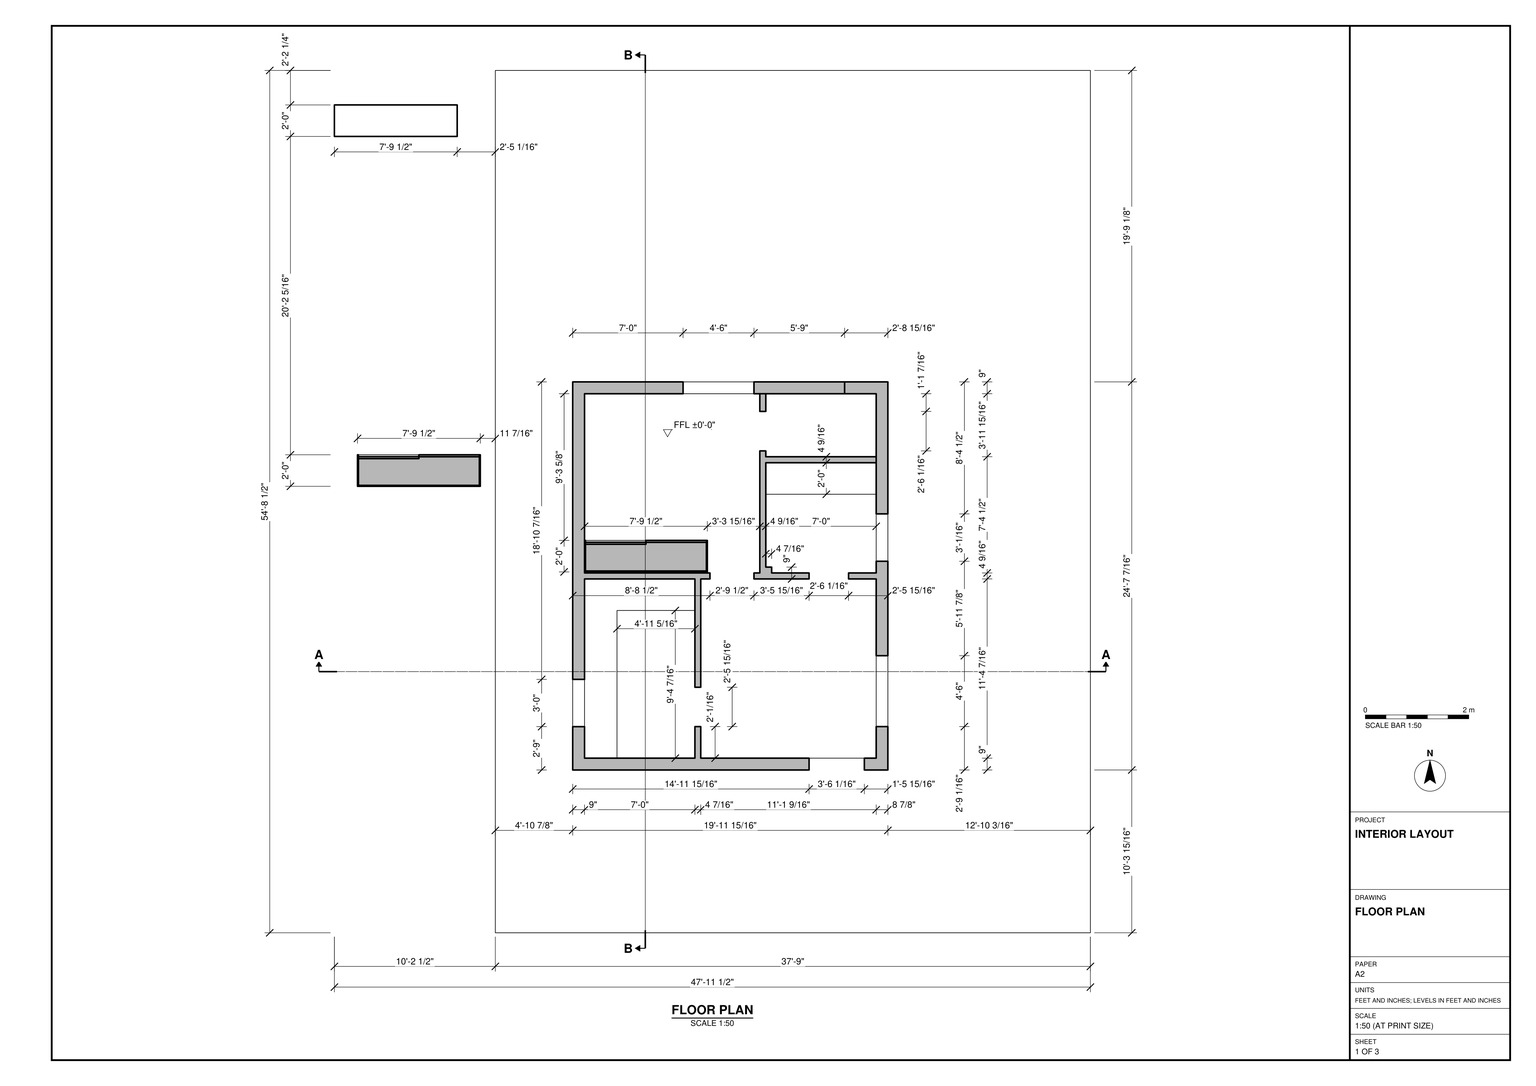
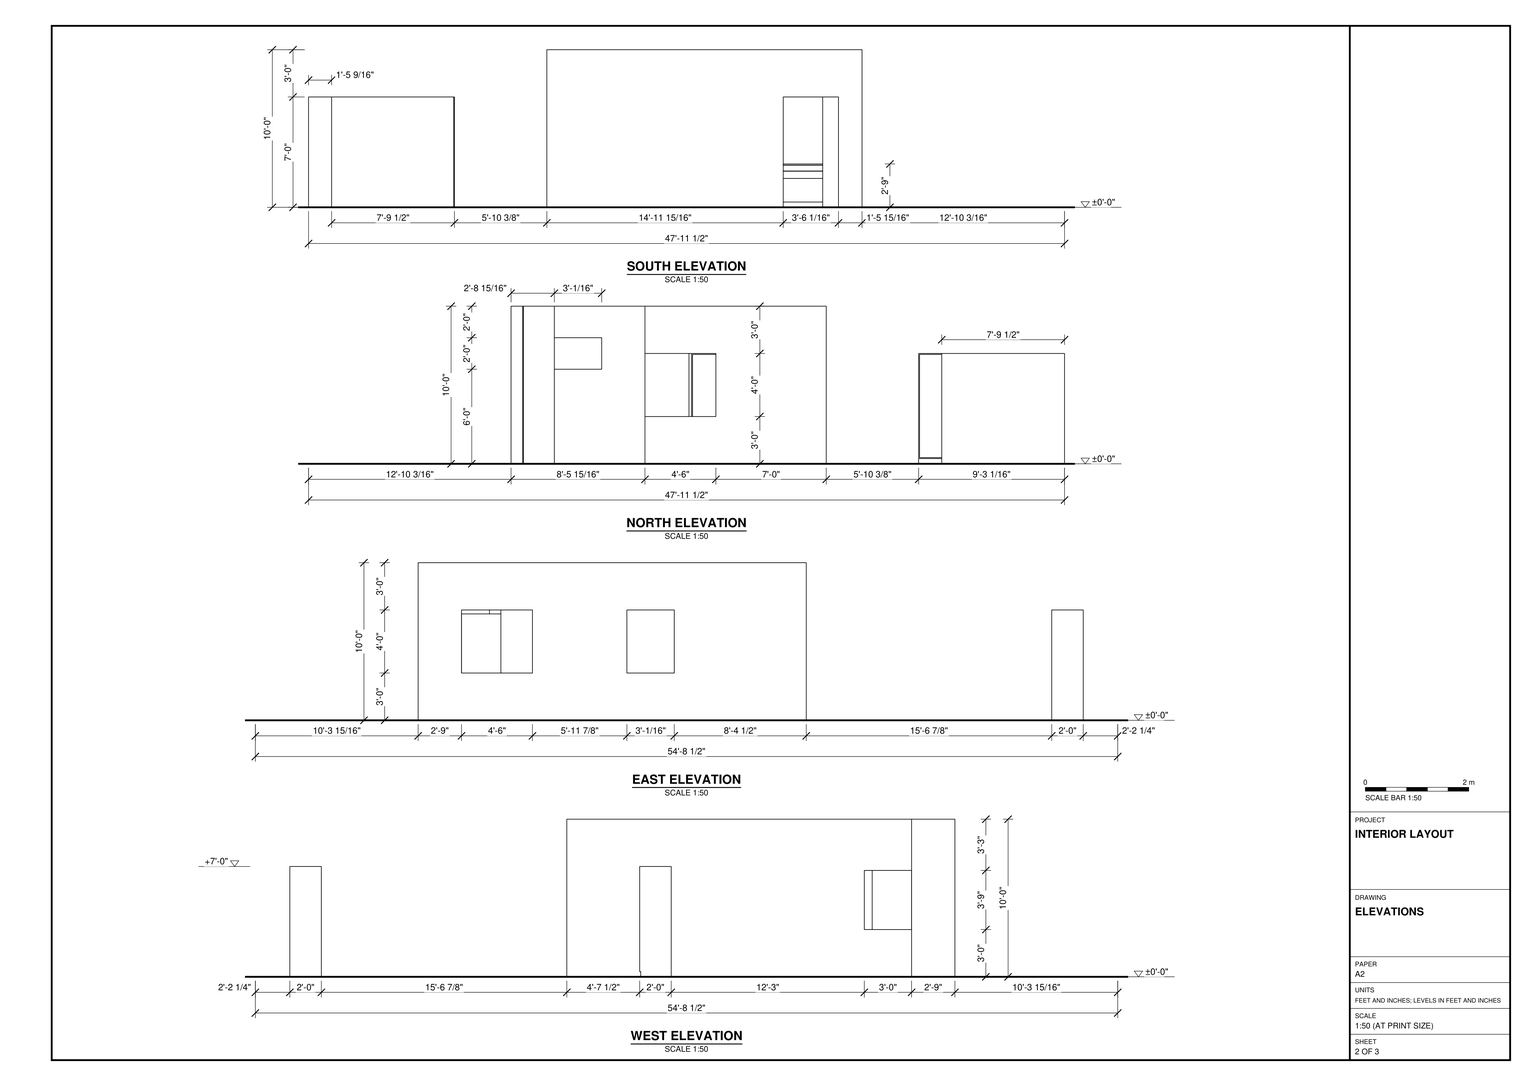
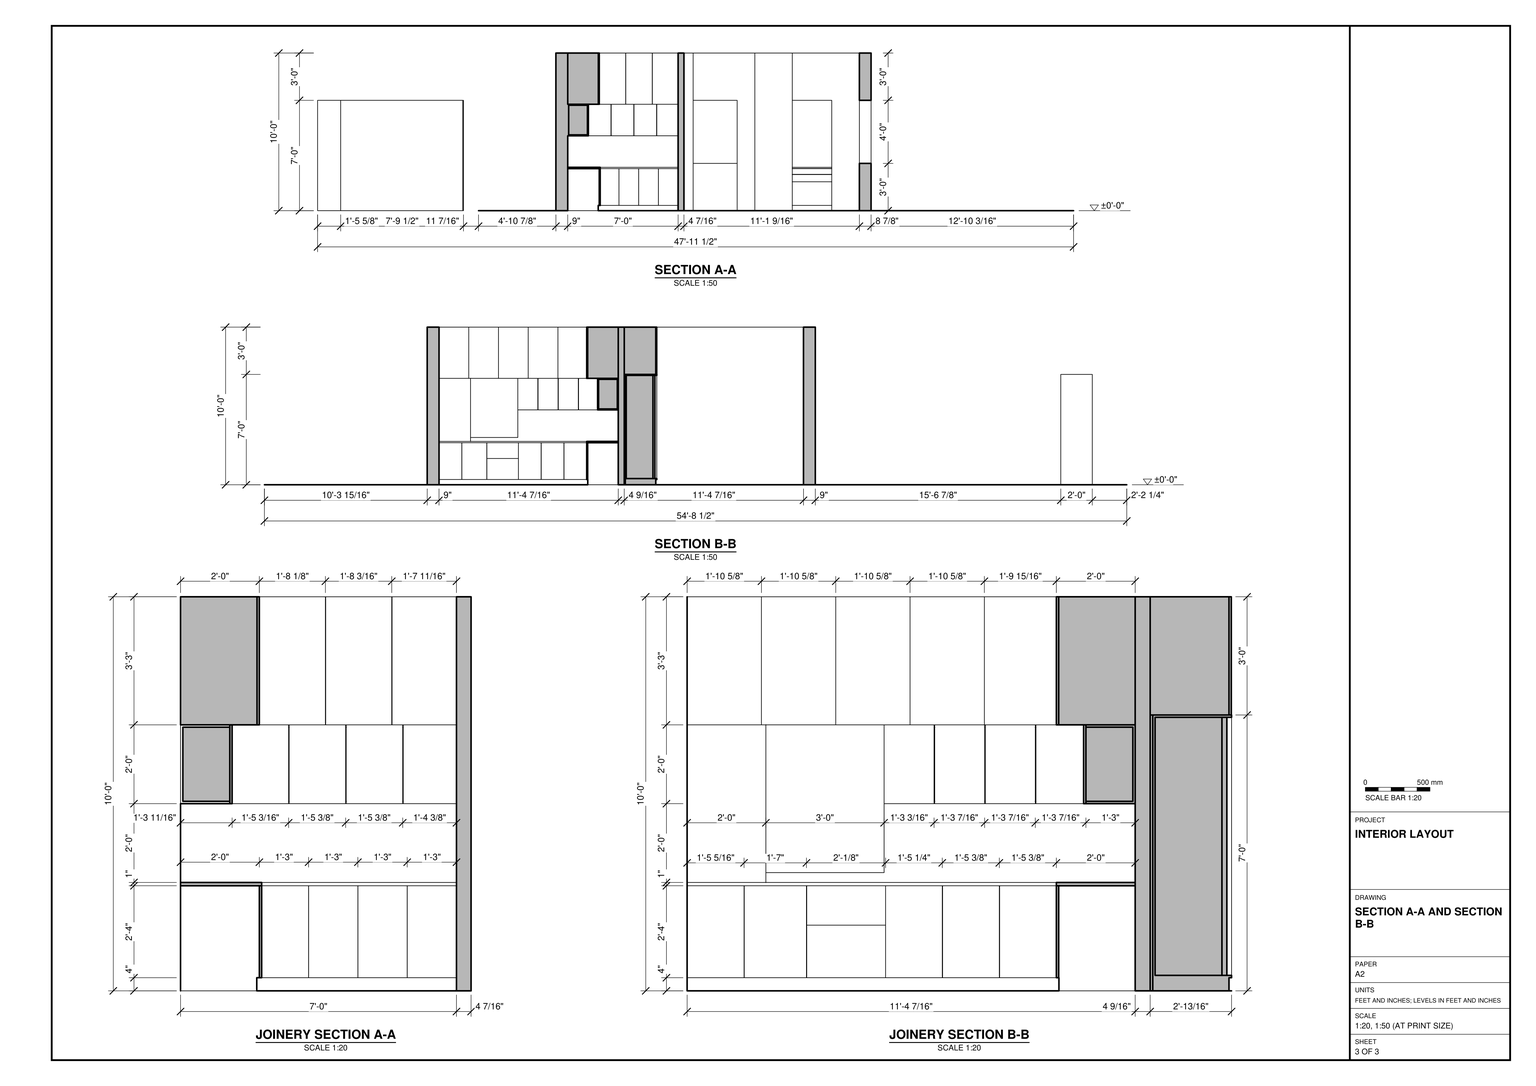
Build the interior layout in SketchUp from task_files/diagram_01.pdf. Work in feet and inches. The complete layout measures 47'-11 1/2" along X by 54'-8 1/2" along Y and is 10'-0" high. Use the single finished floor level of ±0'-0". These overall dimensions include the floor area and the detached units west of it; they are not the dimensions of the room enclosure.

Set out the rectangular floor area, then locate the enclosure using the offsets on the plan. Model the perimeter walls at their drawn thicknesses and the thinner partitions that define the southwest and northeast rooms. Leave the passages between rooms open. Use the elevations to distinguish the floor-level entrance from the window openings and to set each sill and head.

Use both enlarged joinery sections to build the cabinet runs in the southwest room. Match the plinths, divided base cabinets, worktop, clear space above it and two tiers of upper cabinets. Include the tall unit on the other side of the partition and the detached rectangular units at their separate positions west of the floor area. Decor and loose items, if used, may be any suitable library components.

Keep shell elements such as walls and the floor separate from the fit-out. Make each furniture or joinery piece a separate group or component and use components for repeated parts. Save one SketchUp model as output_files/single_storey_interior_with_cabinet_runs.skp.

# SketchUp Ruby script. Lengths in inches.
U = 1.inch
M = Sketchup.active_model
def pt(a) = Geom::Point3d.new(a.map { |v| v * U })
def face(e, loops, mat)
  f = e.add_face(loops[0].map { |a| pt(a) })
  loops[1..].each { |l| e.add_face(l.map { |a| pt(a) }).erase! }
  f.material = f.back_material = mat if mat
  f
end
# faces: each face lists its corners as indices into pts; further lists are holes
def faces(e, pts, list, mat = nil) = list.each { |f| face(e, (f[0].is_a?(Array) ? f : [f]).map { |l| l.map { |i| pts[i] } }, mat) }
# xy, xz, yz: faces in a plane at the given z, y or x. An outline is a flat list of corners, or four numbers for a rectangle; further outlines are holes
def ring(l) = l.size == 4 ? [[l[0], l[1]], [l[2], l[1]], [l[2], l[3]], [l[0], l[3]]] : l.each_slice(2).to_a
def flat(e, list, mat, &to3) = list.each { |f| face(e, (f[0].is_a?(Array) ? f : [f]).map { |l| ring(l).map { |u, v| to3.(u, v) } }, mat) }
def xy(e, z, list, mat = nil) = flat(e, list, mat) { |x, y| [x, y, z] }
def xz(e, y, list, mat = nil) = flat(e, list, mat) { |x, z| [x, y, z] }
def yz(e, x, list, mat = nil) = flat(e, list, mat) { |y, z| [x, y, z] }
def lines(e, pts, list) = list.each { |a, b| e.add_line(pt(pts[a]), pt(pts[b])) }
# prism: a flat outline (further loops are holes) pulled along v
def prism(e, loops, v, mat = nil)
  f = face(e, loops, mat); d = Geom::Vector3d.new(v.map { |x| x * U })
  f.pushpull(f.normal.samedirection?(d) ? d.length : -d.length)
end
def box(e, o, s, mat = nil) = prism(e, [[o, [o[0] + s[0], o[1], o[2]], [o[0] + s[0], o[1] + s[1], o[2]], [o[0], o[1] + s[1], o[2]]]], [0, 0, s[2]], mat)
def at(x, y, z, deg = 0) = Geom::Transformation.translation(pt([x, y, z])) * Geom::Transformation.rotation(ORIGIN, Z_AXIS, deg.degrees)
def axes(o, x, y, z) = Geom::Transformation.new([*x, 0, *y, 0, *z, 0, *pt(o).to_a, 1])
def part(name) = M.definitions.add(name)
# library, detail: a bought-in or finely detailed component or shape, given as its bounding box
def library(name, o, s) = part(name).tap { |d| box(d.entities, o, s) }
def detail(e, o, s) = box(e.add_group.entities, o, s)
def put(e, d, t, mat = nil) = e.add_instance(d, t).tap { |i| i.material = mat if mat }
def group(e, t, mat = nil) = e.add_group.tap { |g| g.transformation = t; g.material = mat if mat }.entities
root = M.entities
M.materials.add("[Color M00]").color = [255, 255, 255]
M.materials.add("[Marble Carrara Floor Tile]").color = [204, 208, 214]
c1 = part("Group\#11")
box(c1.entities,[0,0,-1.42],[0.71,15.21,24])
c2 = part("Group\#2")
box(c2.entities,[0.02,0,0],[14.99,0.71,28],"[Color M00]")
c3 = part("Group\#18")
xy(c3.entities,0,[[0,0,93.47,23.21]],"[Color M00]")
xy(c3.entities,4,[[0,23.21,93.47,24]],"[Color M00]")
xy(c3.entities,4.71,[[0.71,0.71,92.76,0.71,92.76,21,46.74,21,46.74,22.5,92.76,22.5,92.76,24,0.71,24],[46.74,21,92.76,22.5]],"[Color M00]")
xy(c3.entities,83.29,[[0.71,0.71,92.76,24]],"[Color M00]")
xy(c3.entities,84,[[0,0,93.47,24]],"[Color M00]")
xz(c3.entities,0,[[0,0,92.92,84],[92.92,0,93.47,84]],"[Color M00]")
xz(c3.entities,0.71,[[0.71,4.71,92.76,83.29]],"[Color M00]")
xz(c3.entities,23.21,[[0,0,93.47,4]],"[Color M00]")
xz(c3.entities,24,[[[0,4,93.47,84],[0.71,4.71,92.76,83.29]]],"[Color M00]")
yz(c3.entities,0,[[0,0,0,84,24,84,24,4,23.21,4,23.21,0]],"[Color M00]")
yz(c3.entities,0.71,[[0.71,4.71,24,83.29]],"[Color M00]")
yz(c3.entities,92.76,[[0.71,4.71,24,83.29]],"[Color M00]")
yz(c3.entities,93.47,[[0,0,23.21,0,23.21,4,24,4,24,84,0,84]],"[Color M00]")
g1 = group(c3.entities,at(0.71,21.07,4.71))
box(g1,[0,0,0],[46.03,1.5,78.58],"[Color M00]")
g2 = group(c3.entities,at(46.74,22.5,4.71))
box(g2,[0,0,0],[46.03,1.5,78.58],"[Color M00]")
c4 = part("Group\#21")
box(c4.entities,[0,0,0],[23.21,0.71,36],"[Color M00]")
c5 = part("Group\#24")
box(c5.entities,[0,0,0],[17,0.71,28],"[Color M00]")
prism(root,[[[92.92,606.25,0],[0,606.25,0],[0,630.25,0],[93.47,630.25,0],[93.47,606.25,0]]],[0,0,84],"[Color M00]")
xy(root,0,[[[122.51,0,575.51,656.5],[181.41,123.93,181.41,419.4,190.42,419.4,190.42,410.38,265.43,410.38,265.43,419.4,352.34,419.4,352.34,410.38,388.4,410.38,388.4,419.4,421.34,419.4,421.34,123.93,403.43,123.93,403.43,132.95,361.36,132.95,361.36,123.93]],[181.41,123.93,274.45,132.95],[274.45,123.93,278.9,132.95],[278.9,123.93,361.36,132.95],[403.43,123.93,412.44,132.95],
  [412.44,123.93,421.34,156.99],[181.41,132.95,190.42,156.93],[274.45,132.95,278.9,156.99],[181.41,156.93,190.42,192.93],[412.44,156.99,421.34,210.96],
  [274.45,186.92,278.9,269.38],[181.41,192.93,190.42,269.38],[412.44,210.96,421.34,282.84],[181.41,269.38,190.42,419.4],[190.42,269.38,283.34,273.95],
  [319.4,269.38,361.36,269.38,361.36,273.95,332.87,273.95,332.87,278.4,328.42,278.4,328.42,357.85,412.44,357.85,412.44,362.42,328.42,362.42,328.42,366.87,323.85,366.87,323.85,273.95,319.4,273.95],[391.41,269.38,412.44,273.95],[412.44,282.84,421.34,410.38],[323.85,396.92,328.42,410.38],[265.43,410.38,319.4,419.4],
  [319.4,410.38,323.85,419.4],[323.85,410.38,332.87,419.4],[332.87,410.38,352.34,419.4],[388.4,410.38,411.94,419.4],[411.94,410.38,412.44,419.4],
  [412.44,410.38,421.34,419.4]])
xy(root,0,[[213.64,132.95,274.45,132.95,274.45,156.99,278.9,156.99,278.9,132.95,412.44,132.95,412.44,269.38,391.41,269.38,391.41,273.95,412.44,273.95,412.44,335.35,328.42,335.35,328.42,278.4,332.87,278.4,332.87,273.95,361.36,273.95,361.36,269.38,319.4,269.38,319.4,273.95,323.85,273.95,323.85,366.87,328.42,366.87,328.42,362.42,412.44,362.42,412.44,410.38,328.42,410.38,328.42,396.92,323.85,396.92,323.85,410.38,190.42,410.38,190.42,297.95,283.9,297.95,283.9,273.95,283.34,273.95,283.34,269.38,278.9,269.38,278.9,186.92,274.45,186.92,274.45,246.17,213.64,246.17],[190.42,273.95,283.9,297.95]],"[Marble Carrara Floor Tile]")
xy(root,4,[[213.64,132.95,214.42,245.38],[213.64,245.38,213.64,246.17,274.45,246.17,274.45,246.09,214.42,246.09,214.42,245.38],[328.42,335.35,412.44,357.85]],"[Color M00]")
xy(root,4,[[328.42,334.56,345.35,335.35],[345.35,334.56,395.44,335.35],[395.44,334.56,412.44,335.35]],"[Marble Carrara Floor Tile]")
xy(root,32,[[190.42,132.95,190.42,269.38,274.45,269.38,274.45,246.09,214.42,246.09,214.42,132.95],[214.42,132.95,215.13,193.375],[214.42,193.375,215.13,210.71],[214.42,210.71,215.13,228.05],[214.42,228.05,215.13,245.38],
  [214.42,245.38,229.43,246.09],[229.43,245.38,244.4375,246.09],[244.4375,245.38,259.44,246.09],[259.44,245.38,274.45,246.09],[328.42,333.85,345.35,334.56],
  [345.35,333.85,395.44,334.56],[395.44,333.85,412.44,334.56]],"[Color M00]")
xy(root,32,[[328.42,334.56,412.44,357.85]],"[Marble Carrara Floor Tile]")
xy(root,33,[[190.42,132.95,215.13,132.95,215.13,245.38,274.45,245.38,274.45,269.38,190.42,269.38]],"[Color M00]")
xy(root,33,[[328.42,333.85,412.44,357.85]],"[Marble Carrara Floor Tile]")
xy(root,36,[[412.44,156.99,421.34,210.96],[412.44,282.84,421.34,318.9]])
xy(root,84,[[361.36,123.93,403.43,132.95],[274.45,156.99,278.9,186.92],[412.44,156.99,421.34,210.96],[285.9,269.38,319.4,273.95],[361.36,269.38,391.41,273.95],
  [412.44,282.84,421.34,318.9],[323.85,366.87,328.42,396.92]])
xy(root,120,[[181.41,123.93,421.34,123.93,421.34,419.4,388.4,419.4,388.4,410.38,412.44,410.38,412.44,273.95,361.36,273.95,361.36,269.38,412.44,269.38,412.44,132.95,278.9,132.95,278.9,186.92,274.45,186.92,274.45,132.95,190.42,132.95,190.42,156.93,181.41,156.93],[285.9,269.38,332.87,269.38,332.87,278.4,328.42,278.4,328.42,357.85,412.44,357.85,412.44,362.42,328.42,362.42,328.42,410.38,323.85,410.38,323.85,273.95,285.9,273.95],[332.87,269.38,361.36,273.95]])
xz(root,123.93,[[181.41,0,361.36,0,361.36,84,403.43,84,403.43,0,421.34,0,421.34,120,181.41,120]])
xz(root,132.95,[[213.64,0,213.64,4,214.42,4,214.42,32,215.13,32,215.13,33,190.42,33,190.42,120,274.45,120,274.45,0],[278.9,0,361.36,120],[403.43,0,403.43,84,361.36,84,361.36,120,412.44,120,412.44,0]])
xz(root,132.95,[[190.42,0,190.42,32,214.42,32,214.42,4,213.64,4,213.64,0],[190.42,32,215.13,33]],"[Color M00]")
xz(root,156.93,[[181.41,0,190.42,120]])
xz(root,156.99,[[274.45,0,278.9,84],[412.44,36,421.34,84]])
xz(root,186.92,[[274.45,84,278.9,120]])
xz(root,210.96,[[412.44,36,421.34,84]])
xz(root,245.38,[[215.13,32,274.45,33]],"[Color M00]")
xz(root,246.09,[[214.42,4,259.44,32],[259.44,4,274.45,32]],"[Color M00]")
xz(root,246.17,[[213.64,0,274.45,4]],"[Color M00]")
xz(root,269.38,[[319.4,0,332.87,0,332.87,120,285.9,120,285.9,84,319.4,84],[332.87,0,361.36,120],[391.41,0,412.44,0,412.44,120,361.36,120,361.36,84,391.41,84]])
xz(root,269.38,[[190.42,0,274.45,32],[190.42,32,274.45,33]],"[Color M00]")
xz(root,273.95,[[319.4,0,319.4,84,285.9,84,285.9,120,323.85,120,323.85,0],[332.87,0,361.36,120],[391.41,0,391.41,84,361.36,84,361.36,120,412.44,120,412.44,0]])
xz(root,278.4,[[328.42,0,332.87,120]])
xz(root,282.84,[[412.44,36,421.34,84]])
xz(root,318.9,[[412.44,36,421.34,84]])
xz(root,333.85,[[328.42,32,345.35,33],[345.35,32,395.44,33],[395.44,32,412.44,33]],"[Marble Carrara Floor Tile]")
xz(root,334.56,[[328.42,4,345.35,32],[345.35,4,395.44,18],[395.44,4,412.44,32],[345.35,18,395.44,26.01],[345.35,26.01,395.44,32]],"[Color M00]")
xz(root,335.35,[[328.42,0,412.44,4]],"[Marble Carrara Floor Tile]")
xz(root,357.85,[[328.42,33,412.44,120]])
xz(root,357.85,[[328.42,4,412.44,32]],"[Color M00]")
xz(root,357.85,[[328.42,0,412.44,4],[328.42,32,412.44,33]],"[Marble Carrara Floor Tile]")
xz(root,362.42,[[328.42,0,412.44,120]])
xz(root,366.87,[[323.85,0,328.42,84]])
xz(root,396.92,[[323.85,0,328.42,84]])
xz(root,410.38,[[323.85,0,328.42,120],[388.4,0,411.94,120],[411.94,0,412.44,120]])
xz(root,419.4,[[388.4,0,411.94,120],[411.94,0,412.44,120],[412.44,0,421.34,120]])
yz(root,181.41,[[123.93,0,156.93,120]])
yz(root,190.42,[[132.95,33,156.93,120]])
yz(root,190.42,[[132.95,0,156.93,32],[156.93,0,192.93,32],[192.93,0,269.38,32],[132.95,32,156.93,33],[156.93,32,192.93,33],
  [192.93,32,269.38,33]],"[Color M00]")
yz(root,213.64,[[132.95,0,246.17,4]],"[Color M00]")
yz(root,214.42,[[132.95,4,193.375,32],[193.375,4,210.71,32],[210.71,4,228.05,32],[228.05,4,246.09,32]],"[Color M00]")
yz(root,215.13,[[132.95,32,245.38,33]],"[Color M00]")
yz(root,274.45,[[132.95,0,132.95,120,186.92,120,186.92,84,156.99,84,156.99,0]])
yz(root,274.45,[[246.17,0,269.38,0,269.38,32,246.09,32,246.09,4,246.17,4],[245.38,32,269.38,33]],"[Color M00]")
yz(root,278.9,[[132.95,0,156.99,0,156.99,84,186.92,84,186.92,120,132.95,120]])
yz(root,285.9,[[269.38,84,273.95,120]])
yz(root,319.4,[[269.38,0,273.95,84]])
yz(root,323.85,[[273.95,0,273.95,120,410.38,120,410.38,0,396.92,0,396.92,84,366.87,84,366.87,0]])
yz(root,328.42,[[278.4,0,335.35,0,335.35,4,334.56,4,334.56,32,333.85,32,333.85,33,357.85,33,357.85,120,278.4,120],[362.42,0,366.87,0,366.87,84,396.92,84,396.92,0,410.38,0,410.38,120,362.42,120]])
yz(root,328.42,[[334.56,4,357.85,32]],"[Color M00]")
yz(root,328.42,[[335.35,0,357.85,4],[333.85,32,357.85,33]],"[Marble Carrara Floor Tile]")
yz(root,332.87,[[273.95,0,278.4,120]])
yz(root,361.36,[[123.93,0,132.95,84],[269.38,0,273.95,84]])
yz(root,388.4,[[410.38,0,419.4,120]])
yz(root,391.41,[[269.38,0,273.95,84]])
yz(root,403.43,[[123.93,0,132.95,84]])
yz(root,412.44,[[[132.95,0,269.38,120],[156.99,36,210.96,84]],[[273.95,0,273.95,120,357.85,120,357.85,33,333.85,33,333.85,32,334.56,32,334.56,4,335.35,4,335.35,0],[282.84,36,318.9,84]],[357.85,0,362.42,120],[362.42,0,410.38,120]])
yz(root,412.44,[[334.56,4,357.85,32]],"[Color M00]")
yz(root,412.44,[[335.35,0,357.85,4],[333.85,32,357.85,33]],"[Marble Carrara Floor Tile]")
yz(root,421.34,[[[123.93,0,419.4,120],[156.99,36,210.96,84],[282.84,36,318.9,84]]])
g3 = group(root,at(190.42,410.38,0))
xy(g3,0,[[-9.02,-253.45,0,-141],[84.02,-223.46,88.47,-136.43],[-9.02,-141,84.02,-136.43],[88.47,-141,95.47,-136.43],[-9.02,-136.43,0,9.02],
  [0,0,128.98,9.02],[128.98,0,197.98,9.02]])
xy(g3,36,[[-9.02,-253.45,0,-217.45],[75.01,0,128.98,9.02]])
xy(g3,57,[[0,-217.45,0,-141,84.02,-141,84.02,-156,15,-156,15,-217.45]])
xy(g3,57.71,[[0.71,-216.74,15,-216.74,15,-156,83.31,-156,83.31,-141.71,0.71,-141.71]])
xy(g3,72,[[161.92,0,197.98,9.02]])
xy(g3,80.29,[[0.71,-216.74,0.71,-141.71,83.31,-141.71,83.31,-156,15,-156,15,-216.74]])
xy(g3,81,[[0,-277.43,15,-217.45],[15,-277.43,15,-156,84.02,-156,84.02,-164.29,23.29,-164.29,23.29,-277.43],[23.29,-277.43,24,-254.81],[23.29,-254.81,24,-232.18],[-9.02,-253.45,0,-217.45],
  [23.29,-232.18,24,-209.55],[0,-217.45,15,-217.45,15,-156,84.02,-156,84.02,-141,0,-141],[23.29,-209.55,24,-186.92],[23.29,-186.92,24,-164.29]])
xy(g3,84,[[75.01,0,128.98,9.02]])
xy(g3,96,[[161.92,0,197.98,9.02]])
xy(g3,120,[[0,-277.43,23.29,-277.43,23.29,-164.29,84.02,-164.29,84.02,-141,0,-141],[23.29,-277.43,24,-254.81],[23.29,-254.81,24,-232.18],[-9.02,-253.45,0,-253.45,0,-141,84.02,-141,84.02,-223.46,88.47,-223.46,88.47,-141,95.47,-141,95.47,-136.43,0,-136.43,0,0,197.98,0,197.98,9.02,-9.02,9.02],[23.29,-232.18,24,-209.55],
  [23.29,-209.55,24,-186.92],[23.29,-186.92,24,-164.29]])
xz(g3,-277.43,[[0,81,23.29,120],[23.29,81,24,120]])
xz(g3,-254.81,[[23.29,81,24,120]])
xz(g3,-253.45,[[-9.02,0,0,36],[-9.02,81,0,120]])
xz(g3,-232.18,[[23.29,81,24,120]])
xz(g3,-223.46,[[84.02,0,88.47,120]])
xz(g3,-217.45,[[-9.02,36,0,36,0,57,15,57,15,81,-9.02,81]])
xz(g3,-216.74,[[0.71,57.71,15,80.29]])
xz(g3,-209.55,[[23.29,81,24,120]])
xz(g3,-186.92,[[23.29,81,24,120]])
xz(g3,-164.29,[[23.29,81,24,120],[24,81,64.02,120],[64.02,81,84.02,120]])
xz(g3,-156,[[15,57,84.02,57,84.02,81,15,81,15,80.29,83.31,80.29,83.31,57.71,15,57.71]])
xz(g3,-141.71,[[0.71,57.71,83.31,80.29]])
xz(g3,-141,[[0,0,84.02,57],[88.47,0,95.47,120],[0,57,84.02,81],[0,81,84.02,120]])
xz(g3,-136.43,[[0,0,95.47,120]])
xz(g3,0,[[0,0,128.98,0,128.98,36,75.01,36,75.01,84,128.98,84,128.98,0,197.98,0,197.98,72,161.92,72,161.92,96,197.98,96,197.98,120,0,120]])
xz(g3,9.02,[[-9.02,0,-9.02,120,128.98,120,128.98,84,75.01,84,75.01,36,128.98,36,128.98,0],[128.98,0,128.98,120,197.98,120,197.98,96,161.92,96,161.92,72,197.98,72,197.98,0]])
yz(g3,-9.02,[[-253.45,0,-253.45,36,-217.45,36,-217.45,81,-253.45,81,-253.45,120,9.02,120,9.02,0]])
yz(g3,0,[[-253.45,0,-141,0,-141,57,-217.45,57,-217.45,36,-253.45,36],[-136.43,0,0,120],[-156,57,-141,81],[-277.43,81,-253.45,120],[-253.45,81,-141,120]])
yz(g3,0.71,[[-216.74,57.71,-141.71,80.29]])
yz(g3,15,[[-217.45,57,-156,57.71],[-217.45,57.71,-216.74,57.71,-216.74,80.29,-202.09,80.29,-202.09,81,-217.45,81],[-216.74,57.71,-202.09,80.29],[-202.09,80.29,-156,81]])
yz(g3,23.29,[[-277.43,81,-254.81,120],[-254.81,81,-232.18,120],[-232.18,81,-209.55,120],[-209.55,81,-186.92,120],[-186.92,81,-164.29,120]])
yz(g3,24,[[-277.43,81,-254.81,120],[-254.81,81,-232.18,120],[-232.18,81,-209.55,120],[-209.55,81,-186.92,120],[-186.92,81,-164.29,120]])
yz(g3,75.01,[[0,36,9.02,84]])
yz(g3,83.31,[[-156,57.71,-141.71,80.29]])
yz(g3,84.02,[[-223.46,0,-223.46,120,-164.29,120,-164.29,81,-156,81,-156,57,-141,57,-141,0],[-156,57,-141,81],[-164.29,81,-141,120]])
yz(g3,88.47,[[-223.46,0,-141,120]])
yz(g3,95.47,[[-141,0,-136.43,120]])
yz(g3,128.98,[[0,0,9.02,36],[0,36,9.02,84]])
yz(g3,161.92,[[0,72,9.02,96]])
yz(g3,197.98,[[0,0,9.02,72],[0,96,9.02,120]])
put(g3,c1,at(15,-217.45,58.42))
put(g3,c1,at(15,-202.04,58.42))
put(g3,c1,at(15,-186.62,58.42))
put(g3,c1,at(15,-171.21,58.42))
g4 = group(g3,at(68.82,-156,58.42,-90))
box(g4,[0,-1,-1.42],[0.71,16.21,24])
g5 = group(g3,at(51.45,-156,58.42,-90))
box(g5,[0,-1,-1.42],[0.71,17.21,24])
g6 = group(g3,at(34.08,-156,58.42,-90))
box(g6,[0,-1,-1.42],[0.71,17.21,24])
g7 = group(g3,at(16.71,-156,58.42,-90))
box(g7,[0,-1,-1.42],[0.71,17.21,24])
g8 = group(g3,at(64.02,-165,81))
box(g8,[0.4,0,0],[19.61,0.71,39])
g9 = group(g3,at(43.81,-165,81))
box(g9,[0.4,0,0],[20.11,0.71,39])
g10 = group(g3,at(23.6,-165,81))
box(g10,[0.4,0,0],[20.11,0.71,39])
put(root,c2,at(259.44,245.38,4))
put(root,c2,at(244.43,245.38,4))
put(root,c2,at(229.42,245.38,4))
put(root,c2,at(214.4,245.38,4))
g11 = group(root,at(214.42,226.51,4))
prism(g11,[[[0.71,18.87,28],[0.71,1.6,28],[0.71,1.6,0],[0.71,17.33,0],[0.71,18.87,0]]],[-0.71,0,0],"[Color M00]")
g12 = group(root,at(214.42,209.15,4))
prism(g12,[[[0.71,18.87,28],[0.71,1.6,28],[0.71,1.6,0],[0.71,17.33,0],[0.71,18.87,0]]],[-0.71,0,0],"[Color M00]")
g13 = group(root,at(214.42,191.78,4))
prism(g13,[[[0.71,18.87,28],[0.71,1.6,28],[0.71,1.6,0],[0.71,17.33,0],[0.71,18.87,0]]],[-0.71,0,0],"[Color M00]")
g14 = group(root,at(214.42,167.78,4))
prism(g14,[[[0.71,25.6,16],[0.71,1.6,16],[0.71,1.6,0],[0.71,17.33,0],[0.71,25.6,0]]],[-0.71,0,0],"[Color M00]")
g15 = group(root,at(214.42,167.78,20))
prism(g15,[[[0.71,25.6,12],[0.71,1.6,12],[0.71,1.6,0],[0.71,17.33,0],[0.71,25.6,0]]],[-0.71,0,0],"[Color M00]")
g16 = group(root,at(214.42,131.35,4))
prism(g16,[[[0.71,18.93,28],[0.71,1.6,28],[0.71,1.6,0],[0.71,17.33,0],[0.71,18.93,0]]],[-0.71,0,0],"[Color M00]")
g17 = group(root,at(214.42,150.35,4))
prism(g17,[[[0.71,18.93,28],[0.71,0,28],[0.71,0,0],[0.71,17.33,0],[0.71,18.93,0]]],[-0.71,0,0],"[Color M00]")
put(root,c3,at(17.58,339.91,0),"[Color M00]")
put(root,c3,at(190.42,274.73,0))
put(root,c4,at(190.42,297.95,84))
put(root,c4,at(213.84,297.95,84))
put(root,c4,at(237.27,297.95,84))
put(root,c4,at(260.69,297.95,84))
g18 = group(root,at(190.42,273.95,84))
xy(g18,0,[[0,0,93.47,24]],"[Color M00]")
xy(g18,36,[[0,0,93.47,24]],"[Color M00]")
xz(g18,0,[[0,0,92.92,36],[92.92,0,93.47,36]],"[Color M00]")
xz(g18,24,[[0,0,23.37,36],[23.37,0,93.47,36]],"[Color M00]")
yz(g18,0,[[0,0,24,36]],"[Color M00]")
yz(g18,93.47,[[0,0,24,36]],"[Color M00]")
put(root,c5,at(328.42,333.85,4))
put(root,c5,at(395.52,333.85,4))
g19 = group(root,at(345.58,333.85,4))
box(g19,[0,0,0],[49.87,0.71,18],"[Color M00]")
g20 = group(root,at(345.58,333.85,22))
g21 = group(g20,at(0,0,0.51))
box(g21,[0,0,-0.5],[49.87,0.71,5.47],"[Color M00]")
g22 = group(g20,at(0,0,6.14))
box(g22,[0,0,-0.5],[49.87,0.71,4.5],"[Color M00]")
